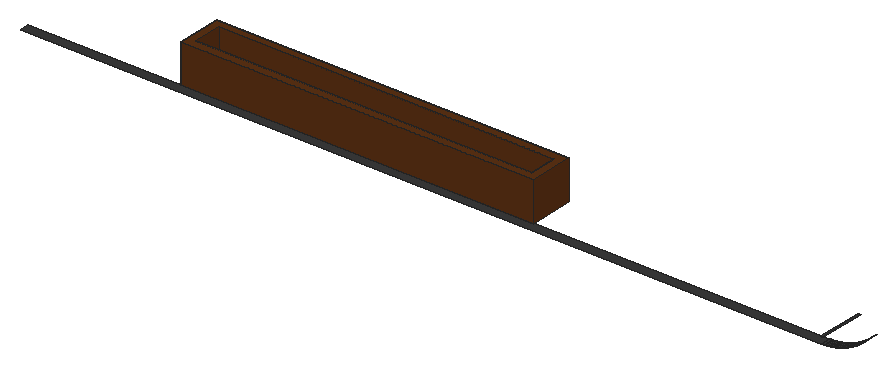
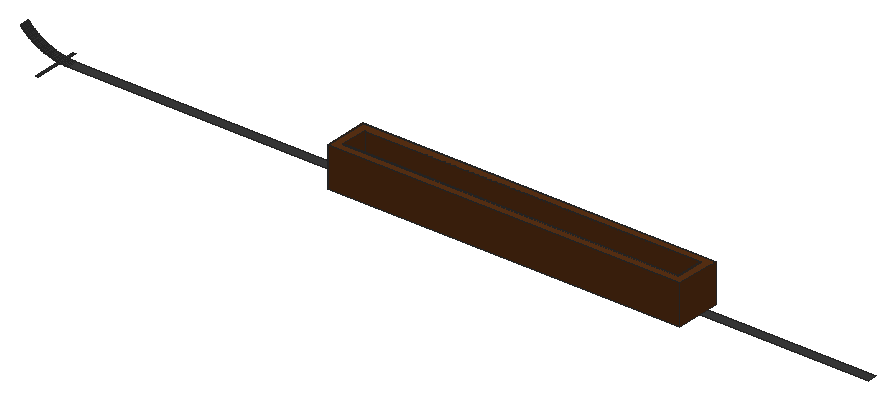
# SketchUp Ruby script. Lengths in inches.
U = 1.inch
M = Sketchup.active_model
def pt(a) = Geom::Point3d.new(a.map { |v| v * U })
def face(e, loops, mat)
  f = e.add_face(loops[0].map { |a| pt(a) })
  loops[1..].each { |l| e.add_face(l.map { |a| pt(a) }).erase! }
  f.material = f.back_material = mat if mat
  f
end
# faces: each face lists its corners as indices into pts; further lists are holes
def faces(e, pts, list, mat = nil) = list.each { |f| face(e, (f[0].is_a?(Array) ? f : [f]).map { |l| l.map { |i| pts[i] } }, mat) }
# xy, xz, yz: faces in a plane at the given z, y or x. An outline is a flat list of corners, or four numbers for a rectangle; further outlines are holes
def ring(l) = l.size == 4 ? [[l[0], l[1]], [l[2], l[1]], [l[2], l[3]], [l[0], l[3]]] : l.each_slice(2).to_a
def flat(e, list, mat, &to3) = list.each { |f| face(e, (f[0].is_a?(Array) ? f : [f]).map { |l| ring(l).map { |u, v| to3.(u, v) } }, mat) }
def xy(e, z, list, mat = nil) = flat(e, list, mat) { |x, y| [x, y, z] }
def xz(e, y, list, mat = nil) = flat(e, list, mat) { |x, z| [x, y, z] }
def yz(e, x, list, mat = nil) = flat(e, list, mat) { |y, z| [x, y, z] }
def lines(e, pts, list) = list.each { |a, b| e.add_line(pt(pts[a]), pt(pts[b])) }
# prism: a flat outline (further loops are holes) pulled along v
def prism(e, loops, v, mat = nil)
  f = face(e, loops, mat); d = Geom::Vector3d.new(v.map { |x| x * U })
  f.pushpull(f.normal.samedirection?(d) ? d.length : -d.length)
end
def box(e, o, s, mat = nil) = prism(e, [[o, [o[0] + s[0], o[1], o[2]], [o[0] + s[0], o[1] + s[1], o[2]], [o[0], o[1] + s[1], o[2]]]], [0, 0, s[2]], mat)
def at(x, y, z, deg = 0) = Geom::Transformation.translation(pt([x, y, z])) * Geom::Transformation.rotation(ORIGIN, Z_AXIS, deg.degrees)
def axes(o, x, y, z) = Geom::Transformation.new([*x, 0, *y, 0, *z, 0, *pt(o).to_a, 1])
def part(name) = M.definitions.add(name)
# library, detail: a bought-in or finely detailed component or shape, given as its bounding box
def library(name, o, s) = part(name).tap { |d| box(d.entities, o, s) }
def detail(e, o, s) = box(e.add_group.entities, o, s)
def put(e, d, t, mat = nil) = e.add_instance(d, t).tap { |i| i.material = mat if mat }
def group(e, t, mat = nil) = e.add_group.tap { |g| g.transformation = t; g.material = mat if mat }.entities
root = M.entities
M.materials.add("1496 AP 8293 CARBON COPY").color = [58, 58, 58]
M.materials.add("[Wood Cherry Original]").color = [91, 49, 20]
xy(root,141,[[46,71,291,74],[291,71,291.26,74]],"1496 AP 8293 CARBON COPY")
xy(root,143,[[291,71,291.24,85]],"1496 AP 8293 CARBON COPY")
xy(root,143.01,[[291.47,71,291.71,85]],"1496 AP 8293 CARBON COPY")
p = [[291.52,71,141.01],[291.26,71,141],[291.26,74,141],[291.52,74,141.01],[291.79,71,141.02],[291.79,74,141.02],
  [292.05,71,141.03],[292.05,74,141.03],[292.31,71,141.04],[292.31,74,141.04],[292.57,71,141.0625],[292.57,74,141.0625],
  [292.83,71,141.08],[292.83,74,141.08],[293.09,71,141.11],[293.09,74,141.11],[293.35,71,141.14],[293.35,74,141.14],
  [293.61,71,141.17],[293.61,74,141.17],[293.87,71,141.21],[293.87,74,141.21],[294.13,71,141.25],[294.13,74,141.25],
  [294.39,71,141.29],[294.39,74,141.29],[294.64,71,141.33],[294.64,74,141.33],[294.9,71,141.38],[294.9,74,141.38],
  [295.16,71,141.4375],[295.16,74,141.4375],[295.41,71,141.49],[295.41,74,141.49],[295.67,71,141.55],[295.67,74,141.55],
  [295.92,71,141.62],[295.92,74,141.62],[296.18,71,141.68],[296.18,74,141.68],[296.43,71,141.75],[296.43,74,141.75],
  [296.68,71,141.82],[296.68,74,141.82],[296.93,71,141.9],[296.93,74,141.9],[297.18,71,141.98],[297.18,74,141.98],
  [297.43,71,142.0625],[297.43,74,142.0625],[297.68,71,142.15],[297.68,74,142.15],[297.92,71,142.24],[297.92,74,142.24],
  [298.17,71,142.33],[298.17,74,142.33],[298.41,71,142.42],[298.41,74,142.42],[298.65,71,142.52],[298.65,74,142.52],
  [298.89,71,142.625],[298.89,74,142.625],[299.13,71,142.73],[299.13,74,142.73],[299.375,71,142.84],[299.375,74,142.84],
  [299.61,71,142.95],[299.61,74,142.95],[299.85,71,143.0625],[299.85,74,143.0625],[291.24,71,143],[291.47,71,143.01],
  [291.47,85,143.01],[291.24,85,143],[291.71,71,143.01],[291.94,71,143.02],[291.94,85,143.02],[291.71,85,143.01],
  [300.08,71,143.18],[300.08,74,143.18],[300.3125,71,143.3],[300.3125,74,143.3],[300.54,71,143.42],[300.54,74,143.42],
  [300.77,71,143.55],[300.77,74,143.55],[301,71,143.68],[301,74,143.68],[301.23,71,143.8125],[301.23,74,143.8125],
  [301.45,71,143.95],[301.45,74,143.95],[301.67,71,144.09],[301.67,74,144.09],[301.89,71,144.23],[301.89,74,144.23],
  [302.11,71,144.37],[302.11,74,144.37],[302.33,71,144.52],[302.33,74,144.52],[302.54,71,144.67],[302.54,74,144.67],
  [302.76,71,144.82],[302.76,74,144.82],[302.97,71,144.97],[302.97,74,144.97],[303.18,71,145.13],[303.18,74,145.13],
  [303.38,71,145.29],[303.38,74,145.29],[303.59,71,145.46],[303.59,74,145.46],[303.79,71,145.625],[303.79,74,145.625],
  [303.99,71,145.79],[303.99,74,145.79],[304.1875,71,145.96],[304.1875,74,145.96],[304.38,71,146.14],[304.38,74,146.14],
  [304.58,71,146.3125],[304.58,74,146.3125],[304.77,71,146.49],[304.77,74,146.49],[304.96,71,146.67],[304.96,74,146.67],
  [305.14,71,146.86],[305.14,74,146.86],[305.33,71,147.04],[305.33,74,147.04],[305.51,71,147.23],[305.51,74,147.23]]
faces(root,p,[[0,1,2,3],[4,0,3,5],[6,4,5,7],[8,6,7,9],[10,8,9,11],[12,10,11,13],[14,12,13,15],[16,14,15,17],
  [18,16,17,19],[20,18,19,21],[22,20,21,23],[24,22,23,25],[26,24,25,27],[28,26,27,29],[30,28,29,31],[32,30,31,33],
  [34,32,33,35],[36,34,35,37],[38,36,37,39],[40,38,39,41],[42,40,41,43],[44,42,43,45],[46,44,45,47],[48,46,47,49],
  [50,48,49,51],[52,50,51,53],[54,52,53,55],[56,54,55,57],[58,56,57,59],[60,58,59,61],[62,60,61,63],[64,62,63,65],
  [66,64,65,67],[68,66,67,69],[70,71,72,73],[74,75,76,77],[78,68,69,79],[80,78,79,81],[82,80,81,83],[84,82,83,85],
  [86,84,85,87],[88,86,87,89],[90,88,89,91],[92,90,91,93],[94,92,93,95],[96,94,95,97],[98,96,97,99],[100,98,99,101],
  [102,100,101,103],[104,102,103,105],[106,104,105,107],[108,106,107,109],[110,108,109,111],[112,110,111,113],[114,112,113,115],[116,114,115,117],
  [118,116,117,119],[120,118,119,121],[122,120,121,123],[124,122,123,125],[126,124,125,127],[128,126,127,129],[130,128,129,131]],"1496 AP 8293 CARBON COPY")
g1 = group(root,at(95.23,75.82,143),"[Wood Cherry Original]")
xy(g1,0,[[0,-4.82,107.77,8.68]])
xy(g1,3,[[2.5,-2.41,105.27,6.27]])
xy(g1,12,[[[0,-4.82,107.77,8.68],[2.5,-2.41,105.27,6.27]]])
xz(g1,-4.82,[[0,0,107.77,12]])
xz(g1,-2.41,[[2.5,3,105.27,12]])
xz(g1,6.27,[[2.5,3,105.27,12]])
xz(g1,8.68,[[0,0,107.77,12]])
yz(g1,0,[[-4.82,0,8.68,12]])
yz(g1,2.5,[[-2.41,3,6.27,12]])
yz(g1,105.27,[[-2.41,3,6.27,12]])
yz(g1,107.77,[[-4.82,0,8.68,12]])
